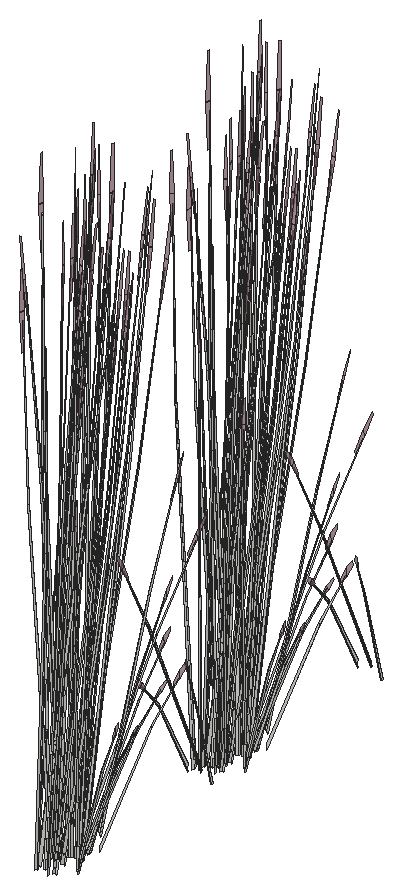
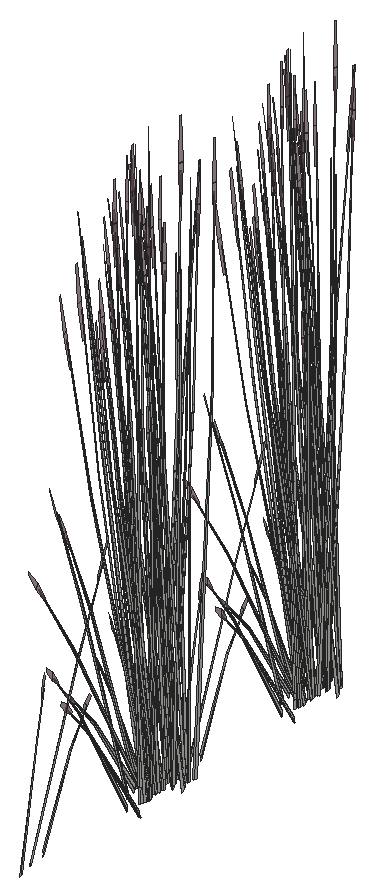
# SketchUp Ruby script. Lengths in inches.
U = 1.inch
M = Sketchup.active_model
def pt(a) = Geom::Point3d.new(a.map { |v| v * U })
def face(e, loops, mat)
  f = e.add_face(loops[0].map { |a| pt(a) })
  loops[1..].each { |l| e.add_face(l.map { |a| pt(a) }).erase! }
  f.material = f.back_material = mat if mat
  f
end
# faces: each face lists its corners as indices into pts; further lists are holes
def faces(e, pts, list, mat = nil) = list.each { |f| face(e, (f[0].is_a?(Array) ? f : [f]).map { |l| l.map { |i| pts[i] } }, mat) }
# xy, xz, yz: faces in a plane at the given z, y or x. An outline is a flat list of corners, or four numbers for a rectangle; further outlines are holes
def ring(l) = l.size == 4 ? [[l[0], l[1]], [l[2], l[1]], [l[2], l[3]], [l[0], l[3]]] : l.each_slice(2).to_a
def flat(e, list, mat, &to3) = list.each { |f| face(e, (f[0].is_a?(Array) ? f : [f]).map { |l| ring(l).map { |u, v| to3.(u, v) } }, mat) }
def xy(e, z, list, mat = nil) = flat(e, list, mat) { |x, y| [x, y, z] }
def xz(e, y, list, mat = nil) = flat(e, list, mat) { |x, z| [x, y, z] }
def yz(e, x, list, mat = nil) = flat(e, list, mat) { |y, z| [x, y, z] }
def lines(e, pts, list) = list.each { |a, b| e.add_line(pt(pts[a]), pt(pts[b])) }
# prism: a flat outline (further loops are holes) pulled along v
def prism(e, loops, v, mat = nil)
  f = face(e, loops, mat); d = Geom::Vector3d.new(v.map { |x| x * U })
  f.pushpull(f.normal.samedirection?(d) ? d.length : -d.length)
end
def box(e, o, s, mat = nil) = prism(e, [[o, [o[0] + s[0], o[1], o[2]], [o[0] + s[0], o[1] + s[1], o[2]], [o[0], o[1] + s[1], o[2]]]], [0, 0, s[2]], mat)
def at(x, y, z, deg = 0) = Geom::Transformation.translation(pt([x, y, z])) * Geom::Transformation.rotation(ORIGIN, Z_AXIS, deg.degrees)
def axes(o, x, y, z) = Geom::Transformation.new([*x, 0, *y, 0, *z, 0, *pt(o).to_a, 1])
def part(name) = M.definitions.add(name)
# library, detail: a bought-in or finely detailed component or shape, given as its bounding box
def library(name, o, s) = part(name).tap { |d| box(d.entities, o, s) }
def detail(e, o, s) = box(e.add_group.entities, o, s)
def put(e, d, t, mat = nil) = e.add_instance(d, t).tap { |i| i.material = mat if mat }
def group(e, t, mat = nil) = e.add_group.tap { |g| g.transformation = t; g.material = mat if mat }.entities
root = M.entities
M.materials.add("LightPink_Translucent").color = [144, 107, 117]
M.materials["LightPink_Translucent"].alpha = 0.75
c1 = part("blade")
p = [[2.15,0.21,22],[0,0.17,0],[0.09,0.45,0],[2.18,0.31,22],[2.29,0.31,22],[0.38,0.45,0],
  [2.48,0.24,33],[2.49,0.24,33],[2.48,0.22,33]]
faces(c1.entities,p,[[0,1,2,3],[4,5,2,3],[6,3,4,7],[8,0,3,6]])
c2 = part("seeds")
p = [[0.3,-0.1,1.38],[-0.01,-0.03,1.59],[-0.01,-0.03,0.03],[0.14,-0.07,-0.07],[0.29,-0.03,3],[0.15,0.01,3.11]]
faces(c2.entities,p,[[0,1,2,3],[1,0,4,5]],"LightPink_Translucent")
c3 = part("blade with seeds")
put(c3.entities,c1,at(0,0,0))
put(c3.entities,c2,axes([2.4,0.25,30.99],[1.5799,-0.05474,1.17369],[-0.12525,1.92788,0.29478],[-0.07173,-0.02425,1.56792]))
put(root,c3,axes([251.73,213.83,0.79],[-0.08351,-0.52716,0],[0.23848,-0.18461,0],[0,0,1.1204]))
put(root,c3,axes([251.43,199.69,0.28],[0.04142,-0.03327,1.27986],[0.24917,0.18313,-0.19552],[0.00729,0.2064,0.218]))
put(root,c3,axes([251.43,214.94,0.28],[0.04142,-0.03327,1.27986],[0.24917,0.18313,-0.19552],[0.00729,0.2064,0.218]))
put(root,c3,axes([252.07,197.54,0.8],[-0.12419,0.55096,-0.32471],[-0.25804,-0.26516,0.15627],[0,0.12701,1.04254]))
put(root,c3,axes([252.07,212.79,0.8],[-0.12419,0.55096,-0.32471],[-0.25804,-0.26516,0.15627],[0,0.12701,1.04254]))
put(root,c3,axes([252.5625,197.21,0.99],[-0.2011,-0.44539,0.12804],[0.20266,-0.432,0.25465],[-0.02221,0.09096,1.1642]))
put(root,c3,axes([252.5625,212.46,0.99],[-0.2011,-0.44539,0.12804],[0.20266,-0.432,0.25465],[-0.02221,0.09096,1.1642]))
put(root,c3,axes([251.87,196.95,0.79],[0,-0.70749,0],[0.32006,0,0],[0,0,1.30246]))
put(root,c3,axes([251.87,212.2,0.79],[0,-0.70749,0],[0.32006,0,0],[0,0,1.30246]))
put(root,c3,axes([251.57,197.08,0.96],[0.28839,0.29636,0.17466],[-0.1388,0.61578,0.36291],[0,-0.14195,1.16519]))
put(root,c3,axes([251.57,212.33,0.96],[0.28839,0.29636,0.17466],[-0.1388,0.61578,0.36291],[0,-0.14195,1.16519]))
put(root,c3,axes([252.03,197.23,0.86],[0,0.70714,-0.04091],[-0.32006,0,0],[0,0.02222,1.30182]))
put(root,c3,axes([252.03,212.48,0.86],[0,0.70714,-0.04091],[-0.32006,0,0],[0,0.02222,1.30182]))
put(root,c3,axes([251.48,196.66,1.17],[-0.27795,0.03775,0.32471],[-0.02514,-0.62656,-0.15627],[0.04976,-0.0635,1.04254]))
put(root,c3,axes([251.48,211.92,1.17],[-0.27795,0.03775,0.32471],[-0.02514,-0.62656,-0.15627],[0.04976,-0.0635,1.04254]))
put(root,c3,axes([251.35,195.59,0.99],[-0.07394,0.60768,0.12804],[-0.27057,-0.17197,0.25465],[0.04674,-0.00296,1.1642]))
put(root,c3,axes([251.35,210.84,0.99],[-0.07394,0.60768,0.12804],[-0.27057,-0.17197,0.25465],[0.04674,-0.00296,1.1642]))
put(root,c3,axes([251.875,198.6,0.86],[0.11128,0.70245,-0.04364],[-0.31797,0.24614,0],[0.00389,0.02453,1.2496]))
put(root,c3,axes([251.875,213.85,0.86],[0.11128,0.70245,-0.04364],[-0.31797,0.24614,0],[0.00389,0.02453,1.2496]))
put(root,c3,axes([251.21,210.09,0.91],[-0.16003,-0.61271,0],[0.26773,-0.34169,-0.37456],[0.06098,-0.07782,1.18819]))
put(root,c3,axes([252.79,197.68,0.79],[-0.3199,-0.00489,-0.03612],[0,-0.68339,0.36248],[-0.01005,0.15557,1.14929]))
put(root,c3,axes([252.79,212.93,0.79],[-0.3199,-0.00489,-0.03612],[0,-0.68339,0.36248],[-0.01005,0.15557,1.14929]))
put(root,c3,axes([252.16,195.62,0.99],[-0.27504,0.16229,0.12804],[-0.06792,-0.60396,0.25465],[0.02453,0.088,1.1642]))
put(root,c3,axes([252.16,210.875,0.99],[-0.27504,0.16229,0.12804],[-0.06792,-0.60396,0.25465],[0.02453,0.088,1.1642]))
put(root,c3,axes([251.88,208.61,1.2],[0.03283,0.35655,0.83364],[-0.18215,-0.19748,0.6125],[0.0196,-0.18257,0.18362]))
put(root,c3,axes([251.88,224.12,1.2],[0.03283,0.35655,0.83364],[-0.18215,-0.19748,0.6125],[0.0196,-0.18257,0.18362]))
put(root,c3,axes([251.71,196.5,0.91],[-0.21222,0.5549,0.33208],[-0.25213,-0.48983,0.13031],[0.05116,-0.05538,1.15295]))
put(root,c3,axes([251.71,211.75,0.91],[-0.21222,0.5549,0.33208],[-0.25213,-0.48983,0.13031],[0.05116,-0.05538,1.15295]))
put(root,c3,axes([252.08,197.38,0.8],[0.17867,0.39495,0],[-0.17867,0.39495,0],[0,0,1.22851]))
put(root,c3,axes([252.08,212.63,0.8],[0.17867,0.39495,0],[-0.17867,0.39495,0],[0,0,1.22851]))
put(root,c3,axes([252.07,196.92,1.17],[0.12419,-0.55096,0.32471],[0.25804,0.26516,-0.15627],[0,0.12701,1.04254]))
put(root,c3,axes([252.07,212.17,1.17],[0.12419,-0.55096,0.32471],[0.25804,0.26516,-0.15627],[0,0.12701,1.04254]))
put(root,c3,axes([251.97,198.83,0.79],[0.25804,0.27452,0],[-0.12419,0.5704,0],[0,0,1.26978]))
put(root,c3,axes([251.97,214.08,0.79],[0.25804,0.27452,0],[-0.12419,0.5704,0],[0,0,1.26978]))
put(root,c3,axes([251.99,196.78,0.92],[-0.32351,-0.12883,0.35707],[0.06584,-0.72759,0.14012],[0.04728,0.07026,1.23973]))
put(root,c3,axes([251.99,212.04,0.92],[-0.32351,-0.12883,0.35707],[0.06584,-0.72759,0.14012],[0.04728,0.07026,1.23973]))
put(root,c3,axes([252.73,197.78,0.66],[-0.17867,0.3815,-0.22483],[-0.17867,-0.3815,0.22483],[0,0.12288,1.00865]))
put(root,c3,axes([252.73,213.03,0.66],[-0.17867,0.3815,-0.22483],[-0.17867,-0.3815,0.22483],[0,0.12288,1.00865]))
put(root,c3,axes([252.22,197.71,0.71],[0.09385,0.55983,-0.50233],[-0.27035,0.20162,-0.13184],[0.01037,0.18957,1.1088]))
put(root,c3,axes([252.22,212.96,0.71],[0.09385,0.55983,-0.50233],[-0.27035,0.20162,-0.13184],[0.01037,0.18957,1.1088]))
put(root,c3,axes([252.08,197.11,0.79],[0.28637,0,0],[0,0.63302,0],[0,0,1.29484]))
put(root,c3,axes([252.08,212.36,0.79],[0.28637,0,0],[0,0.63302,0],[0,0,1.29484]))
put(root,c3,axes([251.81,196.41,1.17],[-0.15376,-0.51322,0.32471],[0.2329,-0.3614,-0.15627],[0.04976,0.0635,1.04254]))
put(root,c3,axes([251.81,211.66,1.17],[-0.15376,-0.51322,0.32471],[0.2329,-0.3614,-0.15627],[0.04976,0.0635,1.04254]))
put(root,c3,axes([251.53,196.53,1.13],[-0.02983,-0.6977,-0.21117],[0.31064,-0.04219,-0.36291],[0.0547,-0.09294,1.15913]))
put(root,c3,axes([251.53,211.78,1.13],[-0.02983,-0.6977,-0.21117],[0.31064,-0.04219,-0.36291],[0.0547,-0.09294,1.15913]))
put(root,c3,axes([252.18,197.04,1.09],[0.23848,-0.17832,0.10509],[0.08351,0.5092,-0.30009],[0,0.11207,0.91989]))
put(root,c3,axes([252.18,212.29,1.09],[0.23848,-0.17832,0.10509],[0.08351,0.5092,-0.30009],[0,0.11207,0.91989]))
put(root,c3,axes([252.1,197.08,1.13],[0.28825,0.29175,-0.21117],[-0.1388,0.61578,-0.36291],[0.00906,0.15119,1.15913]))
put(root,c3,axes([252.1,212.34,1.13],[0.28825,0.29175,-0.21117],[-0.1388,0.61578,-0.36291],[0.00906,0.15119,1.15913]))
put(root,c3,axes([251.49,194.99,0.66],[0.23879,0.15129,-0.22483],[-0.06012,0.53279,0.22483],[0.04814,-0.06144,1.00865]))
put(root,c3,axes([251.49,210.24,0.66],[0.23879,0.15129,-0.22483],[-0.06012,0.53279,0.22483],[0.04814,-0.06144,1.00865]))
put(root,c3,axes([252.15,209.6,1.07],[-0.07276,0.12376,1.03788],[-0.21789,-0.21662,-0.22321],[0.04039,-0.2694,0.44375]))
put(root,c3,axes([252.15,225.11,1.07],[-0.07276,0.12376,1.03788],[-0.21789,-0.21662,-0.22321],[0.04039,-0.2694,0.44375]))
put(root,c3,axes([252.73,197.22,0.99],[0,-0.61145,0.36036],[0.28637,0,0],[0,0.13926,1.14313]))
put(root,c3,axes([252.73,212.48,0.99],[0,-0.61145,0.36036],[0.28637,0,0],[0,0.13926,1.14313]))
put(root,c3,axes([252.85,197.79,0.66],[0,0.61145,-0.36036],[-0.28637,0,0],[0,0.13926,1.14313]))
put(root,c3,axes([252.85,213.04,0.66],[0,0.61145,-0.36036],[-0.28637,0,0],[0,0.13926,1.14313]))
put(root,c3,axes([251.43,210,0.66],[0.23955,-0.30573,-0.36036],[0.14318,0.54821,0],[0.05456,-0.06963,1.14313]))
put(root,c3,axes([251.91,196.26,1.09],[0.04938,-0.54569,0.10509],[0.24125,0.09472,-0.30009],[0.0439,0.05603,0.91989]))
put(root,c3,axes([251.91,211.52,1.09],[0.04938,-0.54569,0.10509],[0.24125,0.09472,-0.30009],[0.0439,0.05603,0.91989]))
put(root,c3,axes([252.25,195.3125,0.99],[-0.23955,-0.30573,0.36036],[0.14318,-0.54821,0],[0.05456,0.06963,1.14313]))
put(root,c3,axes([252.25,210.57,0.99],[-0.23955,-0.30573,0.36036],[0.14318,-0.54821,0],[0.05456,0.06963,1.14313]))
put(root,c3,axes([252.05,198.51,0.78],[0.26872,-0.20746,-0.13933],[0.09442,0.59762,0.00006],[0.02966,-0.02293,1.26212]))
put(root,c3,axes([252.05,213.76,0.78],[0.26872,-0.20746,-0.13933],[0.09442,0.59762,0.00006],[0.02966,-0.02293,1.26212]))
put(root,c3,axes([252.05,196.73,0.8],[0.15376,0.51322,-0.32471],[-0.2329,0.3614,0.15627],[0.04976,0.0635,1.04254]))
put(root,c3,axes([252.05,211.98,0.8],[0.15376,0.51322,-0.32471],[-0.2329,0.3614,0.15627],[0.04976,0.0635,1.04254]))
put(root,c3,axes([252.49,199.06,1.2],[-0.14411,-0.17581,0.83364],[0.18609,-0.17864,0.6125],[0.05019,0.15132,0.18362]))
put(root,c3,axes([252.49,214.3125,1.2],[-0.14411,-0.17581,0.83364],[0.18609,-0.17864,0.6125],[0.05019,0.15132,0.18362]))
put(root,c3,axes([251.97,198.87,1.07],[0.00452,-0.20269,1.03788],[0.21585,-0.22641,-0.22321],[0.06663,0.2426,0.44375]))
put(root,c3,axes([251.97,214.125,1.07],[0.00452,-0.20269,1.03788],[0.21585,-0.22641,-0.22321],[0.06663,0.2426,0.44375]))
put(root,c3,axes([251.71,211.25,0.6875],[0.1724,-0.45959,-0.45255],[0.21416,0.41674,-0.11877],[0.06908,-0.11465,0.99892]))
put(root,c3,axes([252.47,195.59,0.66],[0.06012,0.53279,-0.22483],[-0.23879,0.15129,0.22483],[0.04814,0.06144,1.00865]))
put(root,c3,axes([252.47,210.84,0.66],[0.06012,0.53279,-0.22483],[-0.23879,0.15129,0.22483],[0.04814,0.06144,1.00865]))
put(root,c3,axes([252.92,197.33,0.92],[0.32006,0,0],[0,0.68339,-0.37456],[0,0.15565,1.18819]))
put(root,c3,axes([252.92,212.58,0.92],[0.32006,0,0],[0,0.68339,-0.37456],[0,0.15565,1.18819]))
put(root,c3,axes([251.89,196.44,1.13],[0.25843,-0.40595,-0.21117],[0.17185,0.5736,-0.36291],[0.06376,0.05825,1.15913]))
put(root,c3,axes([251.89,211.69,1.13],[0.25843,-0.40595,-0.21117],[0.17185,0.5736,-0.36291],[0.06376,0.05825,1.15913]))
put(root,c3,axes([252.51,199.86,1.13],[-0.16414,-0.01918,0.76251],[0.10839,-0.40729,0.421],[0.06484,0.1447,0.59812]))
put(root,c3,axes([252.51,215.11,1.13],[-0.16414,-0.01918,0.76251],[0.10839,-0.40729,0.421],[0.06484,0.1447,0.59812]))
put(root,c3,axes([251.23,196.08,0.35],[-0.25194,0.2448,0.93574],[-0.08019,-0.7024,0.36359],[0.1547,0.01169,1.0643]))
put(root,c3,axes([251.23,211.33,0.35],[-0.25194,0.2448,0.93574],[-0.08019,-0.7024,0.36359],[0.1547,0.01169,1.0643]))
put(root,c3,axes([252.39,194.99,0.92],[0.16003,-0.61271,0],[0.26773,0.34169,-0.37456],[0.06098,0.07782,1.18819]))
put(root,c3,axes([252.39,210.25,0.92],[0.16003,-0.61271,0],[0.26773,0.34169,-0.37456],[0.06098,0.07782,1.18819]))
put(root,c3,axes([252.66,209.98,0.28],[-0.03831,-0.04817,1.27986],[-0.0984,-0.53815,-0.19552],[0.06638,-0.14604,0.218]))
put(root,c3,axes([252.66,225.49,0.28],[-0.03831,-0.04817,1.27986],[-0.0984,-0.53815,-0.19552],[0.06638,-0.14604,0.218]))
put(root,c3,axes([252.54,195.36,0.66],[0.23955,0.30573,-0.36036],[-0.14318,0.54821,0],[0.05456,0.06963,1.14313]))
put(root,c3,axes([252.54,210.61,0.66],[0.23955,0.30573,-0.36036],[-0.14318,0.54821,0],[0.05456,0.06963,1.14313]))
put(root,c3,axes([252.53,199.71,0.28],[0.01865,-0.08828,1.27986],[0.23477,-0.25998,-0.19552],[0.07118,0.13456,0.218]))
put(root,c3,axes([252.53,214.96,0.28],[0.01865,-0.08828,1.27986],[0.23477,-0.25998,-0.19552],[0.07118,0.13456,0.218]))
put(root,c3,axes([252.1875,196.53,0.6875],[0.26625,0.10025,-0.45255],[-0.05619,0.61836,-0.11877],[0.07946,0.07493,0.99892]))
put(root,c3,axes([252.1875,211.79,0.6875],[0.26625,0.10025,-0.45255],[-0.05619,0.61836,-0.11877],[0.07946,0.07493,0.99892]))
put(root,c3,axes([253.32,196.9,0.83],[-0.15869,-0.39099,-0.04709],[0.1738,-0.35825,-0.21349],[0.04925,-0.02522,0.70419]))
put(root,c3,axes([253.32,212.15,0.83],[-0.15869,-0.39099,-0.04709],[0.1738,-0.35825,-0.21349],[0.04925,-0.02522,0.70419]))
put(root,c3,axes([252.96,210.16,1.2],[-0.08525,0.31126,0.83364],[-0.07328,-0.41819,0.6125],[0.07041,-0.10479,0.18362]))
put(root,c3,axes([253.36,197.61,1.2],[-0.15814,0.10094,0.83364],[0.07444,-0.41719,0.6125],[0.0839,0.02855,0.18362]))
put(root,c3,axes([253.36,212.87,1.2],[-0.15814,0.10094,0.83364],[0.07444,-0.41719,0.6125],[0.0839,0.02855,0.18362]))
put(root,c3,axes([252.85,211.05,1.07],[-0.09144,-0.01811,1.03788],[-0.09368,-0.48584,-0.22321],[0.11233,-0.13744,0.44375]))
put(root,c3,axes([253.02,197.41,0.63],[-0.16485,0.07338,1.02759],[-0.02624,-0.58408,0.05882],[0.11546,-0.08841,0.58473]))
put(root,c3,axes([253.02,212.67,0.63],[-0.16485,0.07338,1.02759],[-0.02624,-0.58408,0.05882],[0.11546,-0.08841,0.58473]))
put(root,c3,axes([253.2,197.03,0.28],[-0.01338,-0.09283,1.27986],[0.09278,-0.54301,-0.19552],[0.09359,-0.00781,0.218]))
put(root,c3,axes([253.2,212.29,0.28],[-0.01338,-0.09283,1.27986],[0.09278,-0.54301,-0.19552],[0.09359,-0.00781,0.218]))
put(root,c3,axes([253.07,198.28,1.07],[-0.06164,-0.15038,1.03788],[0.0802,-0.49748,-0.22321],[0.12472,0.06739,0.44375]))
put(root,c3,axes([253.07,213.53,1.07],[-0.06164,-0.15038,1.03788],[0.0802,-0.49748,-0.22321],[0.12472,0.06739,0.44375]))
